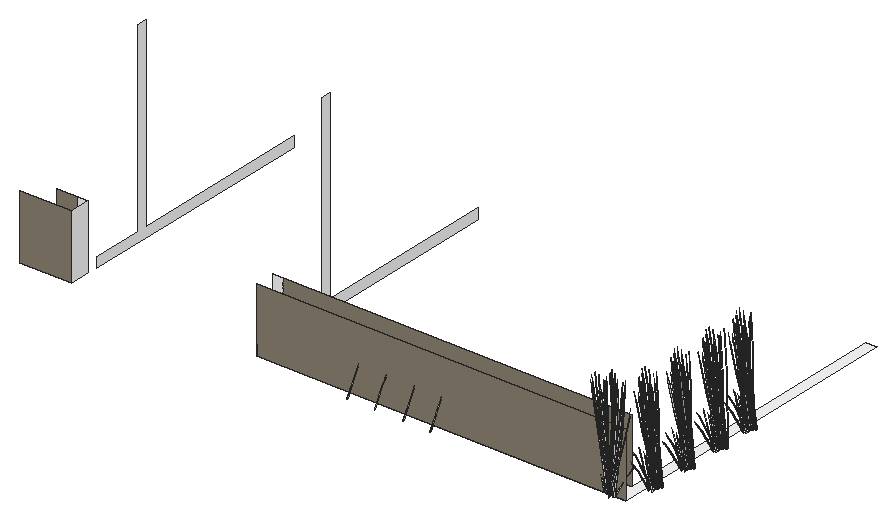
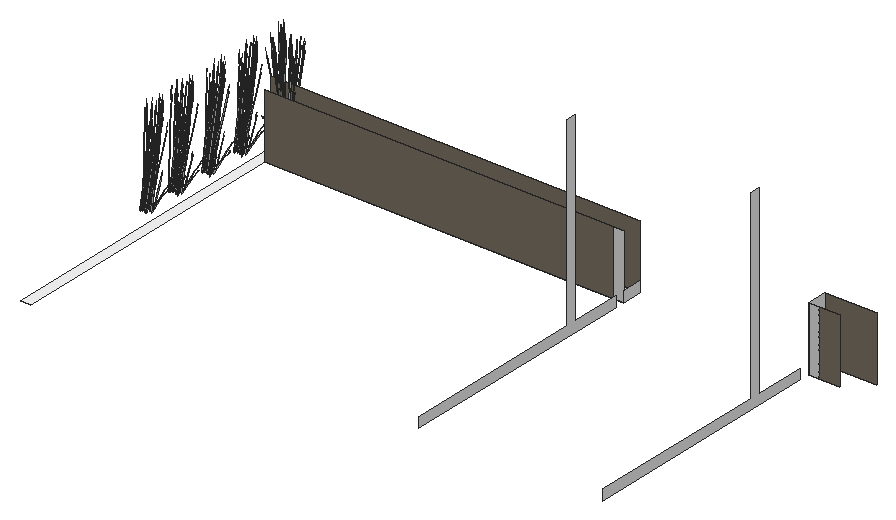
# SketchUp Ruby script. Lengths in inches.
U = 1.inch
M = Sketchup.active_model
def pt(a) = Geom::Point3d.new(a.map { |v| v * U })
def face(e, loops, mat)
  f = e.add_face(loops[0].map { |a| pt(a) })
  loops[1..].each { |l| e.add_face(l.map { |a| pt(a) }).erase! }
  f.material = f.back_material = mat if mat
  f
end
# faces: each face lists its corners as indices into pts; further lists are holes
def faces(e, pts, list, mat = nil) = list.each { |f| face(e, (f[0].is_a?(Array) ? f : [f]).map { |l| l.map { |i| pts[i] } }, mat) }
# xy, xz, yz: faces in a plane at the given z, y or x. An outline is a flat list of corners, or four numbers for a rectangle; further outlines are holes
def ring(l) = l.size == 4 ? [[l[0], l[1]], [l[2], l[1]], [l[2], l[3]], [l[0], l[3]]] : l.each_slice(2).to_a
def flat(e, list, mat, &to3) = list.each { |f| face(e, (f[0].is_a?(Array) ? f : [f]).map { |l| ring(l).map { |u, v| to3.(u, v) } }, mat) }
def xy(e, z, list, mat = nil) = flat(e, list, mat) { |x, y| [x, y, z] }
def xz(e, y, list, mat = nil) = flat(e, list, mat) { |x, z| [x, y, z] }
def yz(e, x, list, mat = nil) = flat(e, list, mat) { |y, z| [x, y, z] }
def lines(e, pts, list) = list.each { |a, b| e.add_line(pt(pts[a]), pt(pts[b])) }
# prism: a flat outline (further loops are holes) pulled along v
def prism(e, loops, v, mat = nil)
  f = face(e, loops, mat); d = Geom::Vector3d.new(v.map { |x| x * U })
  f.pushpull(f.normal.samedirection?(d) ? d.length : -d.length)
end
def box(e, o, s, mat = nil) = prism(e, [[o, [o[0] + s[0], o[1], o[2]], [o[0] + s[0], o[1] + s[1], o[2]], [o[0], o[1] + s[1], o[2]]]], [0, 0, s[2]], mat)
def at(x, y, z, deg = 0) = Geom::Transformation.translation(pt([x, y, z])) * Geom::Transformation.rotation(ORIGIN, Z_AXIS, deg.degrees)
def axes(o, x, y, z) = Geom::Transformation.new([*x, 0, *y, 0, *z, 0, *pt(o).to_a, 1])
def part(name) = M.definitions.add(name)
# library, detail: a bought-in or finely detailed component or shape, given as its bounding box
def library(name, o, s) = part(name).tap { |d| box(d.entities, o, s) }
def detail(e, o, s) = box(e.add_group.entities, o, s)
def put(e, d, t, mat = nil) = e.add_instance(d, t).tap { |i| i.material = mat if mat }
def group(e, t, mat = nil) = e.add_group.tap { |g| g.transformation = t; g.material = mat if mat }.entities
root = M.entities
M.materials.add("LightPink_Translucent").color = [144, 107, 117]
M.materials["LightPink_Translucent"].alpha = 0.75
M.materials.add("M00_Soft_Cloud").color = [255, 255, 255]
M.materials.add("Plaster_04_1K").color = [142, 132, 117]
c1 = part("blade")
p = [[2.15,0.21,22],[0,0.17,0],[0.09,0.45,0],[2.18,0.31,22],[2.29,0.31,22],[0.38,0.45,0],
  [2.48,0.24,33],[2.49,0.24,33],[2.48,0.22,33]]
faces(c1.entities,p,[[0,1,2,3],[4,5,2,3],[6,3,4,7],[8,0,3,6]])
c2 = part("seeds")
p = [[0.3,-0.1,1.38],[-0.01,-0.03,1.59],[-0.01,-0.03,0.03],[0.14,-0.07,-0.07],[0.29,-0.03,3],[0.15,0.01,3.11]]
faces(c2.entities,p,[[0,1,2,3],[1,0,4,5]],"LightPink_Translucent")
c3 = part("blade with seeds")
put(c3.entities,c1,at(0,0,0))
put(c3.entities,c2,axes([2.4,0.25,30.99],[1.5799,-0.05474,1.17369],[-0.12525,1.92788,0.29478],[-0.07173,-0.02425,1.56792]))
xy(root,255,[[186,63.98,402,63.98,402,246.98,396,246.98,396,75.98,186,75.98]],"M00_Soft_Cloud")
xz(root,63.98,[[48,255,78,292.64],[186,255,402,292.64]],"Plaster_04_1K")
xz(root,75.98,[[72,255,78,292.64],[186,255,192,292.64]],"M00_Soft_Cloud")
xz(root,75.98,[[60,255,72,292.64],[192,255,396,292.64]],"Plaster_04_1K")
yz(root,78,[[63.98,255,75.98,292.64],[82.09,255,225.98,255,225.98,261,117.98,261,117.98,369,111.98,369,111.98,261,82.09,261]],"M00_Soft_Cloud")
yz(root,186,[[63.98,255,75.98,261],[82.09,255,82.09,261,111.98,261,111.98,369,117.98,369,117.98,261,225.98,261,225.98,255]],"M00_Soft_Cloud")
put(root,c3,axes([245.1,56.2,256.49],[0.12297,-0.03325,1.76342],[0.73967,0.18301,-0.26939],[0.02163,0.20626,0.30037]))
put(root,c3,axes([261.16,56.2,256.49],[0.12297,-0.03325,1.76342],[0.73967,0.18301,-0.26939],[0.02163,0.20626,0.30037]))
put(root,c3,axes([277.89,56.2,256.49],[0.12297,-0.03325,1.76342],[0.73967,0.18301,-0.26939],[0.02163,0.20626,0.30037]))
put(root,c3,axes([293.62,56.2,256.49],[0.12297,-0.03325,1.76342],[0.73967,0.18301,-0.26939],[0.02163,0.20626,0.30037]))
put(root,c3,axes([390.49,62.375,256.49],[0.10192,0.06105,1.76342],[0.17281,0.56562,-0.26939],[-0.22588,0.12062,0.30037]))
put(root,c3,axes([392.63,62.09,257.375],[-0.47504,0.61229,0],[-0.79476,-0.34146,-0.51607],[-0.18101,-0.07777,1.63711]))
put(root,c3,axes([394.13,60.64,257.67],[-0.76714,0.40567,-0.29095],[-0.51013,-0.57321,-0.50002],[-0.18927,-0.05821,1.59708]))
put(root,c3,axes([394.64,61.09,257.06],[-0.51177,0.45928,-0.62353],[-0.63575,-0.41646,-0.16365],[-0.20507,0.11457,1.37633]))
put(root,c3,axes([394.99,60.83,257.46],[-0.74193,-0.49181,-0.25192],[0.6243,-0.55226,0.5513],[-0.19979,0.05753,1.68216]))
put(root,c3,axes([394.62,60.72,257.21],[-0.82508,0.03772,-0.44739],[-0.07462,-0.62614,0.21531],[-0.14771,0.06346,1.43643]))
put(root,c3,axes([395.48,62.34,257.02],[-0.7111,0.30552,-0.49651],[-0.42504,-0.54784,0],[-0.16196,0.06958,1.57504]))
put(root,c3,axes([395.53,62.17,257.19],[-0.46912,-0.61443,-0.05142],[0.79476,-0.34146,0.51607],[-0.19584,0.0585,1.6363]))
put(root,c3,axes([395.32,62.1,257.03],[-0.70886,-0.15119,-0.30978],[0.17848,-0.53243,0.30978],[-0.1429,0.0614,1.38974]))
put(root,c3,axes([395.19,60.55,257.67],[0.08854,0.69723,-0.29095],[-0.92215,0.04216,-0.50002],[-0.16238,0.09287,1.59708]))
put(root,c3,axes([394.36,61.56,257.2],[-0.76598,-0.27433,0],[0.36864,-0.57001,0],[0,0,1.62707]))
put(root,c3,axes([396.13,62.24,257.375],[0.47504,0.61229,0],[-0.79476,0.34146,-0.51607],[-0.18101,0.07777,1.63711]))
put(root,c3,axes([395.55,61.86,257.33],[0.95122,0.19861,0.30756],[-0.23797,0.7099,-0.36492],[-0.15744,0.08885,1.64885]))
put(root,c3,axes([394.53,61.32,257.2],[-0.24791,-0.5268,0],[0.70791,-0.18448,0],[0,0,1.54371]))
put(root,c3,axes([393.63,62.43,256.49],[0.12297,-0.03325,1.76342],[0.73967,0.18301,-0.26939],[0.02163,0.20626,0.30037]))
put(root,c3,axes([395.53,60.28,257.21],[-0.36864,0.55059,-0.44739],[-0.76598,-0.26498,0.21531],[0,0.12692,1.43643]))
put(root,c3,axes([395.4,59.97,257.29],[0,0.70667,-0.05637],[-0.95008,0,0],[0,0.02221,1.79368]))
put(root,c3,axes([394.95,61.34,257.29],[0.33034,0.70197,-0.06012],[-0.94388,0.24598,0],[0.01154,0.02451,1.72173]))
put(root,c3,axes([397.68,60.42,257.2],[-0.94962,-0.00489,-0.04976],[0,-0.68292,0.49943],[-0.02984,0.15546,1.58352]))
put(root,c3,axes([395.55,60.12,257.21],[0.53038,0.39469,0],[-0.53038,0.39469,0],[0,0,1.69266]))
put(root,c3,axes([395.23,61.57,257.2],[0.76598,0.27433,0],[-0.36864,0.57001,0],[0,0,1.74954]))
put(root,c3,axes([397.48,60.52,257.03],[-0.53038,0.38124,-0.30978],[-0.53038,-0.38124,0.30978],[0,0.1228,1.38974]))
put(root,c3,axes([395.97,60.45,257.09],[0.2786,0.55945,-0.69212],[-0.80253,0.20149,-0.18165],[0.03079,0.18945,1.52773]))
put(root,c3,axes([395.57,59.85,257.21],[0.85008,0,0],[0,0.63259,0],[0,0,1.78407]))
put(root,c3,axes([395.625,59.82,257.67],[0.85568,0.29155,-0.29095],[-0.41201,0.61537,-0.50002],[0.02689,0.15109,1.59708]))
put(root,c3,axes([397.84,60.53,257.02],[0,0.61104,-0.49651],[-0.85008,0,0],[0,0.13917,1.57504]))
put(root,c3,axes([395.46,61.24,257.18],[0.79769,-0.20732,-0.19198],[0.2803,0.59721,0.00008],[0.08805,-0.02292,1.73897]))
put(root,c3,axes([395.47,59.47,257.21],[0.45644,0.51287,-0.44739],[-0.69137,0.36116,0.21531],[0.14771,0.06346,1.43643]))
put(root,c3,axes([396.72,58.33,257.03],[0.17848,0.53243,-0.30978],[-0.70886,0.15119,0.30978],[0.1429,0.0614,1.38974]))
put(root,c3,axes([398.06,60.07,257.375],[0.95008,0,0],[0,0.68292,-0.51607],[0,0.15554,1.63711]))
put(root,c3,axes([404.9375,147.43,256.49],[0.01927,0.0963,1.76342],[-0.38846,0.5029,-0.26939],[-0.27592,-0.02535,0.30037]))
put(root,c3,axes([405.22,125.02,256.49],[0.01927,0.0963,1.76342],[-0.38846,0.5029,-0.26939],[-0.27592,-0.02535,0.30037]))
put(root,c3,axes([405.31,78.11,256.49],[0.01927,0.0963,1.76342],[-0.38846,0.5029,-0.26939],[-0.27592,-0.02535,0.30037]))
put(root,c3,axes([405.43,101.64,256.49],[0.01927,0.0963,1.76342],[-0.38846,0.5029,-0.26939],[-0.27592,-0.02535,0.30037]))
put(root,c3,axes([396.89,62.45,256.49],[0.05536,-0.08822,1.76342],[0.69692,-0.25981,-0.26939],[0.21129,0.13447,0.30037]))
put(root,c3,axes([405.01,127.72,256.49],[0.10192,0.06105,1.76342],[0.17281,0.56562,-0.26939],[-0.22588,0.12062,0.30037]))
put(root,c3,axes([405.1,80.81,256.49],[0.10192,0.06105,1.76342],[0.17281,0.56562,-0.26939],[-0.22588,0.12062,0.30037]))
put(root,c3,axes([395.88,59.27,257.06],[0.79037,0.10018,-0.62353],[-0.16679,0.61794,-0.16365],[0.23587,0.07488,1.37633]))
put(root,c3,axes([405.23,104.33,256.49],[0.10192,0.06105,1.76342],[0.17281,0.56562,-0.26939],[-0.22588,0.12062,0.30037]))
put(root,c3,axes([407.48,148.31,257.06],[-0.79037,-0.10018,-0.62353],[0.16679,-0.61794,-0.16365],[-0.23587,-0.07488,1.37633]))
put(root,c3,axes([407.76,125.9,257.06],[-0.79037,-0.10018,-0.62353],[0.16679,-0.61794,-0.16365],[-0.23587,-0.07488,1.37633]))
put(root,c3,axes([407.85,78.98,257.06],[-0.79037,-0.10018,-0.62353],[0.16679,-0.61794,-0.16365],[-0.23587,-0.07488,1.37633]))
put(root,c3,axes([406.44,149.48,257.02],[-0.7111,-0.30552,-0.49651],[0.42504,-0.54784,0],[-0.16196,-0.06958,1.57504]))
put(root,c3,axes([407.98,102.51,257.06],[-0.79037,-0.10018,-0.62353],[0.16679,-0.61794,-0.16365],[-0.23587,-0.07488,1.37633]))
put(root,c3,axes([406.13,144.93,256.49],[-0.0736,0.08049,1.76342],[-0.74378,0.17355,-0.26939],[-0.17968,-0.15788,0.30037]))
put(root,c3,axes([406.875,149.85,257.375],[-0.47504,0.61229,0],[-0.79476,-0.34146,-0.51607],[-0.18101,-0.07777,1.63711]))
put(root,c3,axes([406.72,127.07,257.02],[-0.7111,-0.30552,-0.49651],[0.42504,-0.54784,0],[-0.16196,-0.06958,1.57504]))
put(root,c3,axes([406.41,122.52,256.49],[-0.0736,0.08049,1.76342],[-0.74378,0.17355,-0.26939],[-0.17968,-0.15788,0.30037]))
put(root,c3,axes([406.8125,80.15,257.02],[-0.7111,-0.30552,-0.49651],[0.42504,-0.54784,0],[-0.16196,-0.06958,1.57504]))
put(root,c3,axes([406.5,75.6,256.49],[-0.0736,0.08049,1.76342],[-0.74378,0.17355,-0.26939],[-0.17968,-0.15788,0.30037]))
put(root,c3,axes([407.15,127.4375,257.375],[-0.47504,0.61229,0],[-0.79476,-0.34146,-0.51607],[-0.18101,-0.07777,1.63711]))
put(root,c3,axes([406.9375,103.68,257.02],[-0.7111,-0.30552,-0.49651],[0.42504,-0.54784,0],[-0.16196,-0.06958,1.57504]))
put(root,c3,axes([406.625,99.13,256.49],[-0.0736,0.08049,1.76342],[-0.74378,0.17355,-0.26939],[-0.17968,-0.15788,0.30037]))
put(root,c3,axes([407.25,80.52,257.375],[-0.47504,0.61229,0],[-0.79476,-0.34146,-0.51607],[-0.18101,-0.07777,1.63711]))
put(root,c3,axes([407.37,104.05,257.375],[-0.47504,0.61229,0],[-0.79476,-0.34146,-0.51607],[-0.18101,-0.07777,1.63711]))
put(root,c3,axes([405.67,145.24,257.13],[-0.21918,0.49894,-0.03893],[-0.6746,-0.15348,-0.17649],[-0.10242,-0.08161,0.58215]))
put(root,c3,axes([405.95,122.83,257.13],[-0.21918,0.49894,-0.03893],[-0.6746,-0.15348,-0.17649],[-0.10242,-0.08161,0.58215]))
put(root,c3,axes([406.04,75.91,257.13],[-0.21918,0.49894,-0.03893],[-0.6746,-0.15348,-0.17649],[-0.10242,-0.08161,0.58215]))
put(root,c3,axes([408.375,148.4,257.67],[-0.76714,0.40567,-0.29095],[-0.51013,-0.57321,-0.50002],[-0.18927,-0.05821,1.59708]))
put(root,c3,axes([406.16,99.44,257.13],[-0.21918,0.49894,-0.03893],[-0.6746,-0.15348,-0.17649],[-0.10242,-0.08161,0.58215]))
put(root,c3,axes([405.31,147.51,257.375],[-0.95008,0,0],[0,-0.68292,-0.51607],[0,-0.15554,1.63711]))
put(root,c3,axes([406.64,149.25,257.03],[-0.17848,-0.53243,-0.30978],[0.70886,-0.15119,0.30978],[-0.1429,-0.0614,1.38974]))
put(root,c3,axes([408.65,125.99,257.67],[-0.76714,0.40567,-0.29095],[-0.51013,-0.57321,-0.50002],[-0.18927,-0.05821,1.59708]))
put(root,c3,axes([408.75,79.08,257.67],[-0.76714,0.40567,-0.29095],[-0.51013,-0.57321,-0.50002],[-0.18927,-0.05821,1.59708]))
put(root,c3,axes([405.58,125.1,257.375],[-0.95008,0,0],[0,-0.68292,-0.51607],[0,-0.15554,1.63711]))
put(root,c3,axes([406.92,126.84,257.03],[-0.17848,-0.53243,-0.30978],[0.70886,-0.15119,0.30978],[-0.1429,-0.0614,1.38974]))
put(root,c3,axes([408.87,102.6,257.67],[-0.76714,0.40567,-0.29095],[-0.51013,-0.57321,-0.50002],[-0.18927,-0.05821,1.59708]))
put(root,c3,axes([405.68,78.19,257.375],[-0.95008,0,0],[0,-0.68292,-0.51607],[0,-0.15554,1.63711]))
put(root,c3,axes([407.01,79.93,257.03],[-0.17848,-0.53243,-0.30978],[0.70886,-0.15119,0.30978],[-0.1429,-0.0614,1.38974]))
put(root,c3,axes([406.04,147.33,257.33],[-0.70674,0.51372,0.30756],[-0.70717,-0.50832,-0.36492],[-0.02468,-0.14589,1.64885]))
put(root,c3,axes([405.8,101.72,257.375],[-0.95008,0,0],[0,-0.68292,-0.51607],[0,-0.15554,1.63711]))
put(root,c3,axes([407.14,103.45,257.03],[-0.17848,-0.53243,-0.30978],[0.70886,-0.15119,0.30978],[-0.1429,-0.0614,1.38974]))
put(root,c3,axes([409.16,126.43,257.06],[-0.51177,0.45928,-0.62353],[-0.63575,-0.41646,-0.16365],[-0.20507,0.11457,1.37633]))
put(root,c3,axes([409.26,79.52,257.06],[-0.51177,0.45928,-0.62353],[-0.63575,-0.41646,-0.16365],[-0.20507,0.11457,1.37633]))
put(root,c3,axes([409.24,148.58,257.46],[-0.74193,-0.49181,-0.25192],[0.6243,-0.55226,0.5513],[-0.19979,0.05753,1.68216]))
put(root,c3,axes([407.89,148.11,257.21],[-0.45644,-0.51287,-0.44739],[0.69137,-0.36116,0.21531],[-0.14771,-0.06346,1.43643]))
put(root,c3,axes([406.32,124.92,257.33],[-0.70674,0.51372,0.30756],[-0.70717,-0.50832,-0.36492],[-0.02468,-0.14589,1.64885]))
put(root,c3,axes([409.38,103.05,257.06],[-0.51177,0.45928,-0.62353],[-0.63575,-0.41646,-0.16365],[-0.20507,0.11457,1.37633]))
put(root,c3,axes([406.41,78.01,257.33],[-0.70674,0.51372,0.30756],[-0.70717,-0.50832,-0.36492],[-0.02468,-0.14589,1.64885]))
put(root,c3,axes([406.54,101.54,257.33],[-0.70674,0.51372,0.30756],[-0.70717,-0.50832,-0.36492],[-0.02468,-0.14589,1.64885]))
put(root,c3,axes([409.52,126.17,257.46],[-0.74193,-0.49181,-0.25192],[0.6243,-0.55226,0.5513],[-0.19979,0.05753,1.68216]))
put(root,c3,axes([408.17,125.7,257.21],[-0.45644,-0.51287,-0.44739],[0.69137,-0.36116,0.21531],[-0.14771,-0.06346,1.43643]))
put(root,c3,axes([408.86,148.48,257.21],[-0.82508,0.03772,-0.44739],[-0.07462,-0.62614,0.21531],[-0.14771,0.06346,1.43643]))
put(root,c3,axes([409.61,79.26,257.46],[-0.74193,-0.49181,-0.25192],[0.6243,-0.55226,0.5513],[-0.19979,0.05753,1.68216]))
put(root,c3,axes([408.26,78.79,257.21],[-0.45644,-0.51287,-0.44739],[0.69137,-0.36116,0.21531],[-0.14771,-0.06346,1.43643]))
put(root,c3,axes([409.73,102.79,257.46],[-0.74193,-0.49181,-0.25192],[0.6243,-0.55226,0.5513],[-0.19979,0.05753,1.68216]))
put(root,c3,axes([408.39,102.3125,257.21],[-0.45644,-0.51287,-0.44739],[0.69137,-0.36116,0.21531],[-0.14771,-0.06346,1.43643]))
put(root,c3,axes([409.14,126.07,257.21],[-0.82508,0.03772,-0.44739],[-0.07462,-0.62614,0.21531],[-0.14771,0.06346,1.43643]))
put(root,c3,axes([409.23,79.16,257.21],[-0.82508,0.03772,-0.44739],[-0.07462,-0.62614,0.21531],[-0.14771,0.06346,1.43643]))
put(root,c3,axes([407.96,148.41,257.4375],[0.20138,-0.72405,-0.23429],[0.95485,0.12621,0.51271],[-0.16685,-0.09999,1.5644]))
put(root,c3,axes([409.36,102.68,257.21],[-0.82508,0.03772,-0.44739],[-0.07462,-0.62614,0.21531],[-0.14771,0.06346,1.43643]))
put(root,c3,axes([405.52,147.05,257.02],[0,-0.61104,-0.49651],[0.85008,0,0],[0,-0.13917,1.57504]))
put(root,c3,axes([408.23,126,257.4375],[0.20138,-0.72405,-0.23429],[0.95485,0.12621,0.51271],[-0.16685,-0.09999,1.5644]))
put(root,c3,axes([409.78,149.93,257.19],[-0.46912,-0.61443,-0.05142],[0.79476,-0.34146,0.51607],[-0.19584,0.0585,1.6363]))
put(root,c3,axes([408.33,79.08,257.4375],[0.20138,-0.72405,-0.23429],[0.95485,0.12621,0.51271],[-0.16685,-0.09999,1.5644]))
put(root,c3,axes([408.45,102.61,257.4375],[0.20138,-0.72405,-0.23429],[0.95485,0.12621,0.51271],[-0.16685,-0.09999,1.5644]))
put(root,c3,axes([410.01,127.69,257.02],[-0.7111,0.30552,-0.49651],[-0.42504,-0.54784,0],[-0.16196,0.06958,1.57504]))
put(root,c3,axes([405.8,124.64,257.02],[0,-0.61104,-0.49651],[0.85008,0,0],[0,-0.13917,1.57504]))
put(root,c3,axes([409.5625,149.85,257.03],[-0.70886,-0.15119,-0.30978],[0.17848,-0.53243,0.30978],[-0.1429,0.0614,1.38974]))
put(root,c3,axes([410.05,127.52,257.19],[-0.46912,-0.61443,-0.05142],[0.79476,-0.34146,0.51607],[-0.19584,0.0585,1.6363]))
put(root,c3,axes([410.1,80.77,257.02],[-0.7111,0.30552,-0.49651],[-0.42504,-0.54784,0],[-0.16196,0.06958,1.57504]))
put(root,c3,axes([405.89,77.73,257.02],[0,-0.61104,-0.49651],[0.85008,0,0],[0,-0.13917,1.57504]))
put(root,c3,axes([410.15,80.61,257.19],[-0.46912,-0.61443,-0.05142],[0.79476,-0.34146,0.51607],[-0.19584,0.0585,1.6363]))
put(root,c3,axes([407.74,147.76,257.67],[-0.85568,-0.29155,-0.29095],[0.41201,-0.61537,-0.50002],[-0.02689,-0.15109,1.59708]))
put(root,c3,axes([410.22,104.3,257.02],[-0.7111,0.30552,-0.49651],[-0.42504,-0.54784,0],[-0.16196,0.06958,1.57504]))
put(root,c3,axes([406.01,101.25,257.02],[0,-0.61104,-0.49651],[0.85008,0,0],[0,-0.13917,1.57504]))
put(root,c3,axes([410.27,104.13,257.19],[-0.46912,-0.61443,-0.05142],[0.79476,-0.34146,0.51607],[-0.19584,0.0585,1.6363]))
put(root,c3,axes([409.84,127.44,257.03],[-0.70886,-0.15119,-0.30978],[0.17848,-0.53243,0.30978],[-0.1429,0.0614,1.38974]))
put(root,c3,axes([409.93,80.53,257.03],[-0.70886,-0.15119,-0.30978],[0.17848,-0.53243,0.30978],[-0.1429,0.0614,1.38974]))
put(root,c3,axes([408.02,125.35,257.67],[-0.85568,-0.29155,-0.29095],[0.41201,-0.61537,-0.50002],[-0.02689,-0.15109,1.59708]))
put(root,c3,axes([409.44,148.31,257.67],[0.08854,0.69723,-0.29095],[-0.92215,0.04216,-0.50002],[-0.16238,0.09287,1.59708]))
put(root,c3,axes([407.36,147.14,257.1],[-0.31203,-0.62659,-0.69835],[0.89884,-0.22566,-0.18329],[-0.03449,-0.21218,1.54149]))
put(root,c3,axes([408.11,78.44,257.67],[-0.85568,-0.29155,-0.29095],[0.41201,-0.61537,-0.50002],[-0.02689,-0.15109,1.59708]))
put(root,c3,axes([410.06,104.06,257.03],[-0.70886,-0.15119,-0.30978],[0.17848,-0.53243,0.30978],[-0.1429,0.0614,1.38974]))
put(root,c3,axes([408.24,101.96,257.67],[-0.85568,-0.29155,-0.29095],[0.41201,-0.61537,-0.50002],[-0.02689,-0.15109,1.59708]))
put(root,c3,axes([409.72,125.9,257.67],[0.08854,0.69723,-0.29095],[-0.92215,0.04216,-0.50002],[-0.16238,0.09287,1.59708]))
put(root,c3,axes([407.64,124.73,257.1],[-0.31203,-0.62659,-0.69835],[0.89884,-0.22566,-0.18329],[-0.03449,-0.21218,1.54149]))
put(root,c3,axes([405.88,147.0625,257.03],[0.53038,-0.38124,-0.30978],[0.53038,0.38124,0.30978],[0,-0.1228,1.38974]))
put(root,c3,axes([408.28,144.6,257.13],[-0.52505,0.35054,-0.03893],[-0.48109,-0.38392,-0.17649],[-0.03387,-0.10878,0.58215]))
put(root,c3,axes([409.8125,78.99,257.67],[0.08854,0.69723,-0.29095],[-0.92215,0.04216,-0.50002],[-0.16238,0.09287,1.59708]))
put(root,c3,axes([407.73,77.82,257.1],[-0.31203,-0.62659,-0.69835],[0.89884,-0.22566,-0.18329],[-0.03449,-0.21218,1.54149]))
put(root,c3,axes([408.07,148.06,257.36],[0.96033,0.12874,0.45755],[-0.19544,0.7271,0.17955],[-0.14034,-0.07021,1.58856]))
put(root,c3,axes([409.9375,102.51,257.67],[0.08854,0.69723,-0.29095],[-0.92215,0.04216,-0.50002],[-0.16238,0.09287,1.59708]))
put(root,c3,axes([407.85,101.34,257.1],[-0.31203,-0.62659,-0.69835],[0.89884,-0.22566,-0.18329],[-0.03449,-0.21218,1.54149]))
put(root,c3,axes([406.16,124.65,257.03],[0.53038,-0.38124,-0.30978],[0.53038,0.38124,0.30978],[0,-0.1228,1.38974]))
put(root,c3,axes([408.56,122.1875,257.13],[-0.52505,0.35054,-0.03893],[-0.48109,-0.38392,-0.17649],[-0.03387,-0.10878,0.58215]))
put(root,c3,axes([406.25,77.74,257.03],[0.53038,-0.38124,-0.30978],[0.53038,0.38124,0.30978],[0,-0.1228,1.38974]))
put(root,c3,axes([408.34,125.65,257.36],[0.96033,0.12874,0.45755],[-0.19544,0.7271,0.17955],[-0.14034,-0.07021,1.58856]))
put(root,c3,axes([408.65,75.28,257.13],[-0.52505,0.35054,-0.03893],[-0.48109,-0.38392,-0.17649],[-0.03387,-0.10878,0.58215]))
put(root,c3,axes([408.4375,78.73,257.36],[0.96033,0.12874,0.45755],[-0.19544,0.7271,0.17955],[-0.14034,-0.07021,1.58856]))
put(root,c3,axes([406.38,101.27,257.03],[0.53038,-0.38124,-0.30978],[0.53038,0.38124,0.30978],[0,-0.1228,1.38974]))
put(root,c3,axes([408.77,98.8,257.13],[-0.52505,0.35054,-0.03893],[-0.48109,-0.38392,-0.17649],[-0.03387,-0.10878,0.58215]))
put(root,c3,axes([408.5625,102.26,257.36],[0.96033,0.12874,0.45755],[-0.19544,0.7271,0.17955],[-0.14034,-0.07021,1.58856]))
put(root,c3,axes([408.6,149.3125,257.2],[-0.76598,-0.27433,0],[0.36864,-0.57001,0],[0,0,1.62707]))
put(root,c3,axes([408.88,126.9,257.2],[-0.76598,-0.27433,0],[0.36864,-0.57001,0],[0,0,1.62707]))
put(root,c3,axes([410.65,127.59,257.375],[0.47504,0.61229,0],[-0.79476,0.34146,-0.51607],[-0.18101,0.07777,1.63711]))
